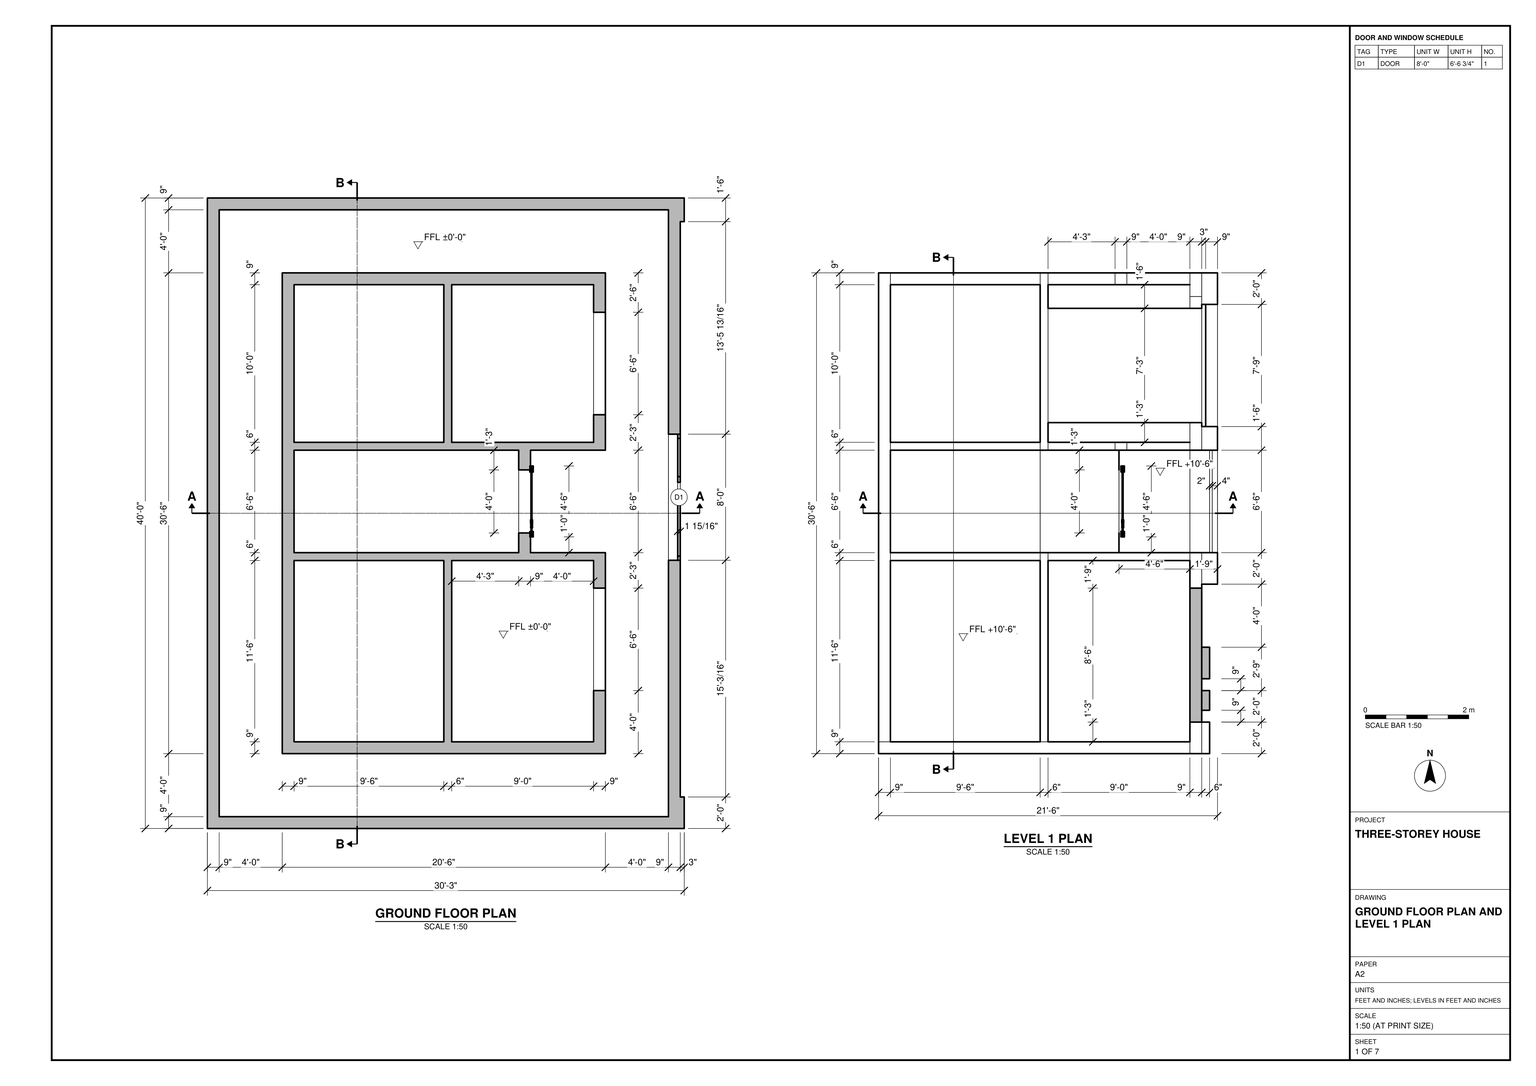
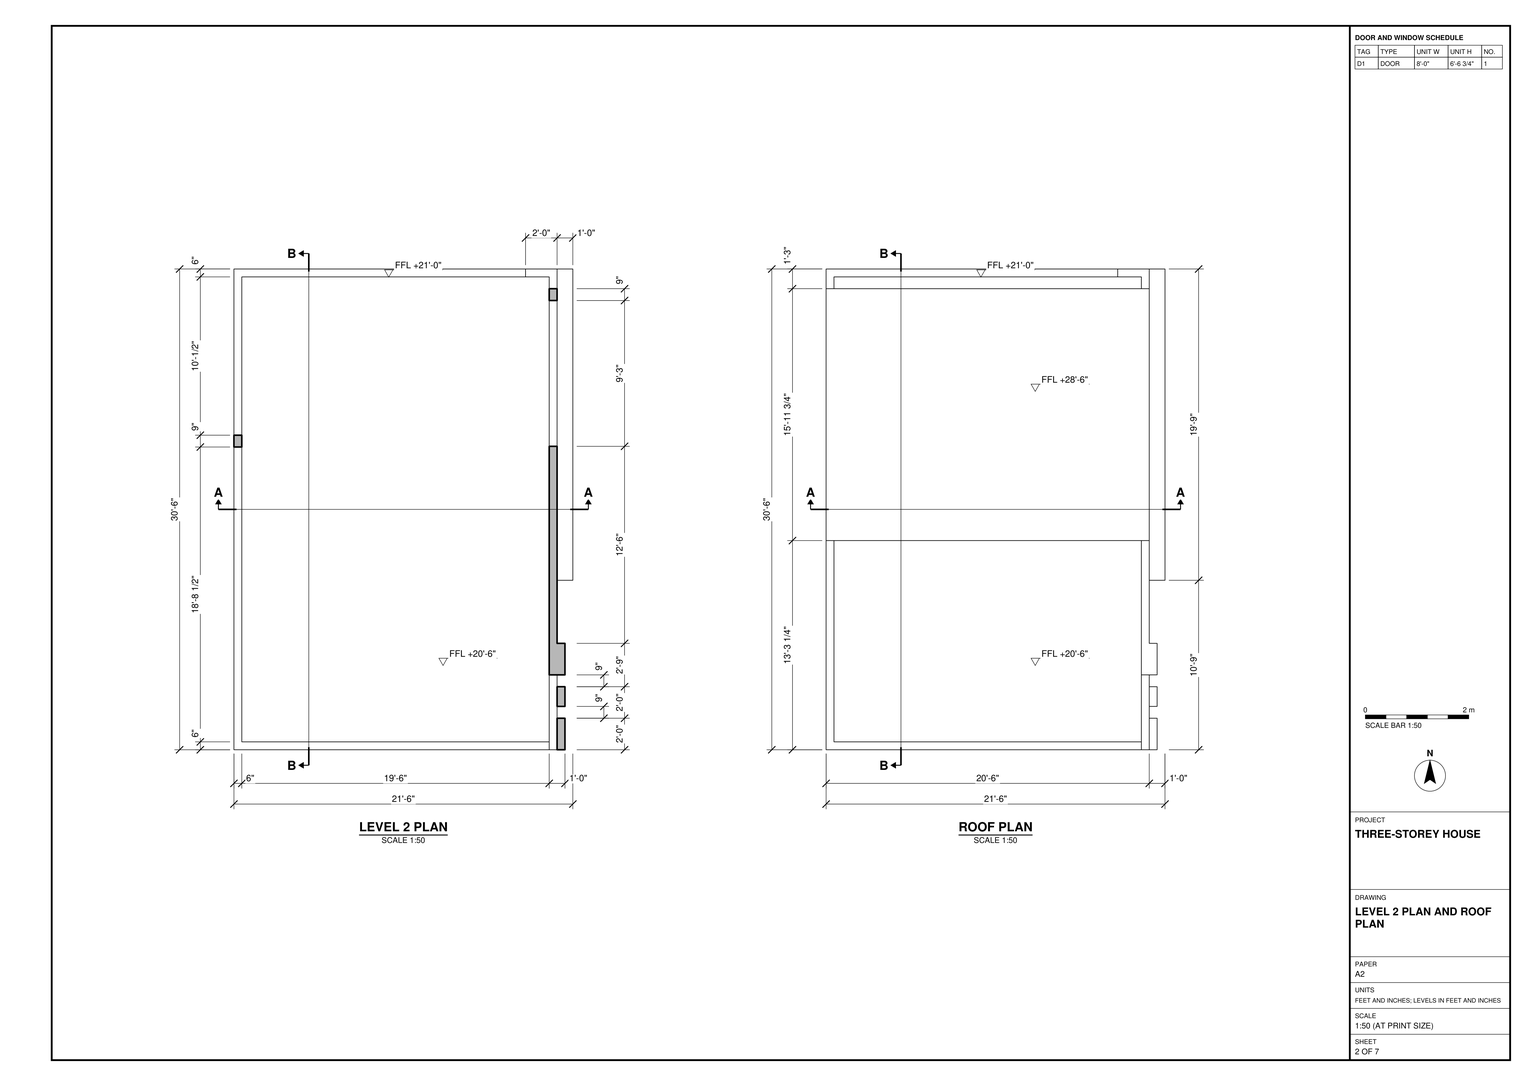
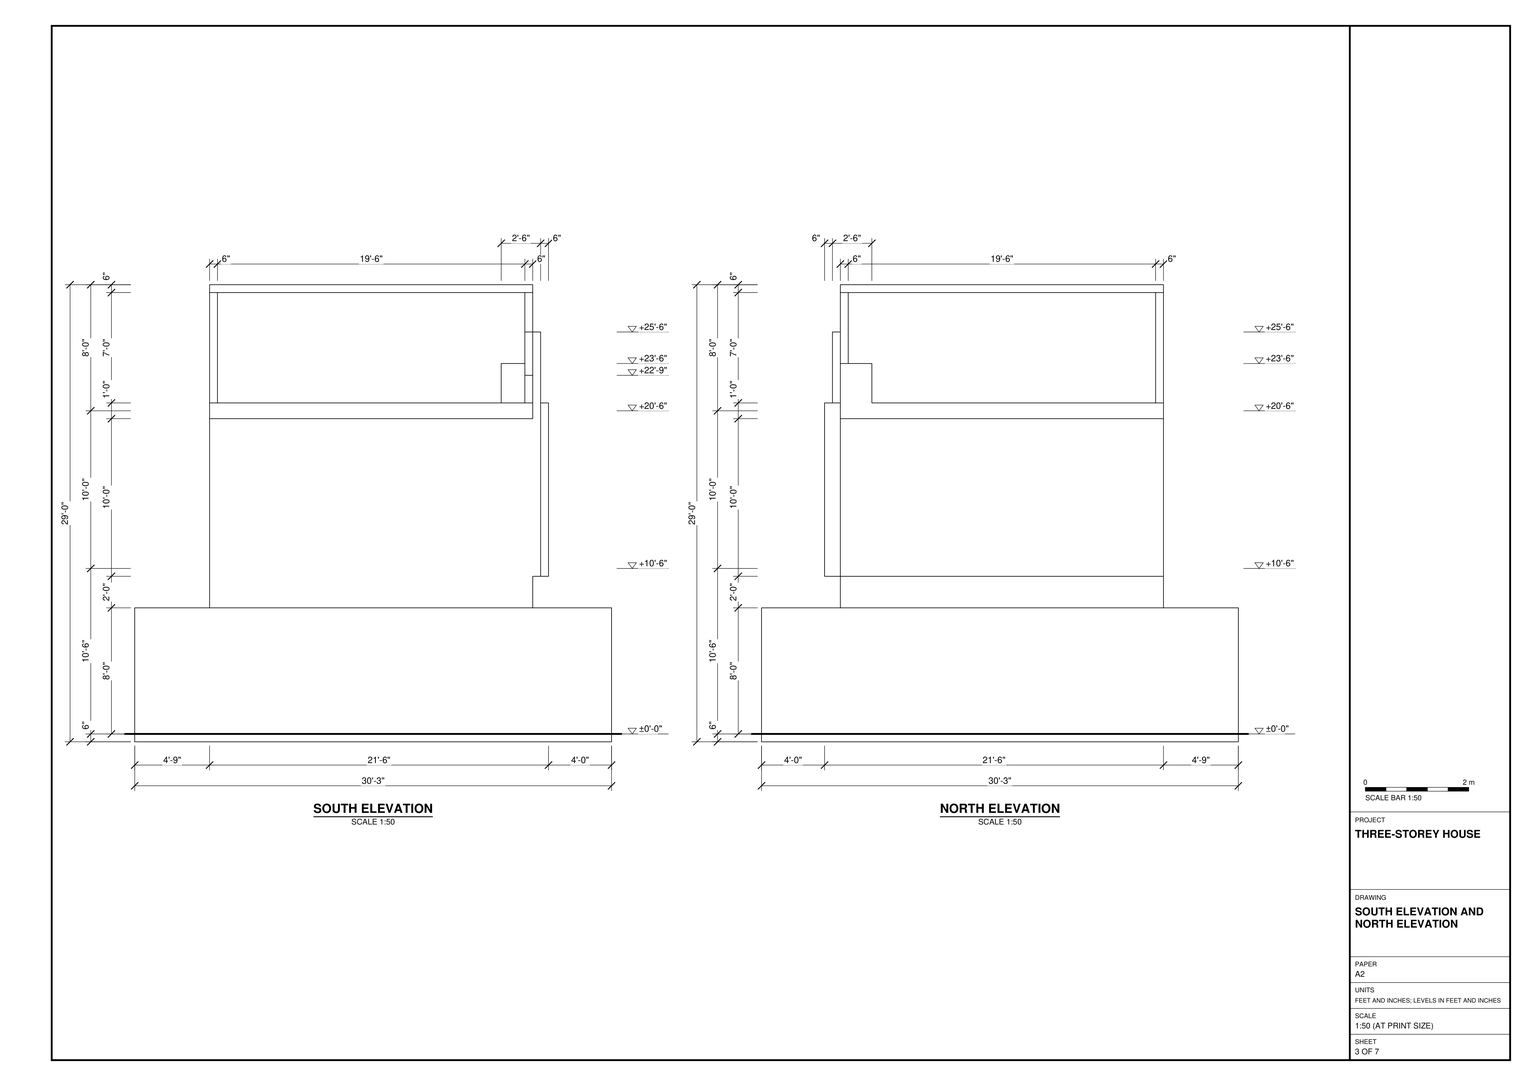
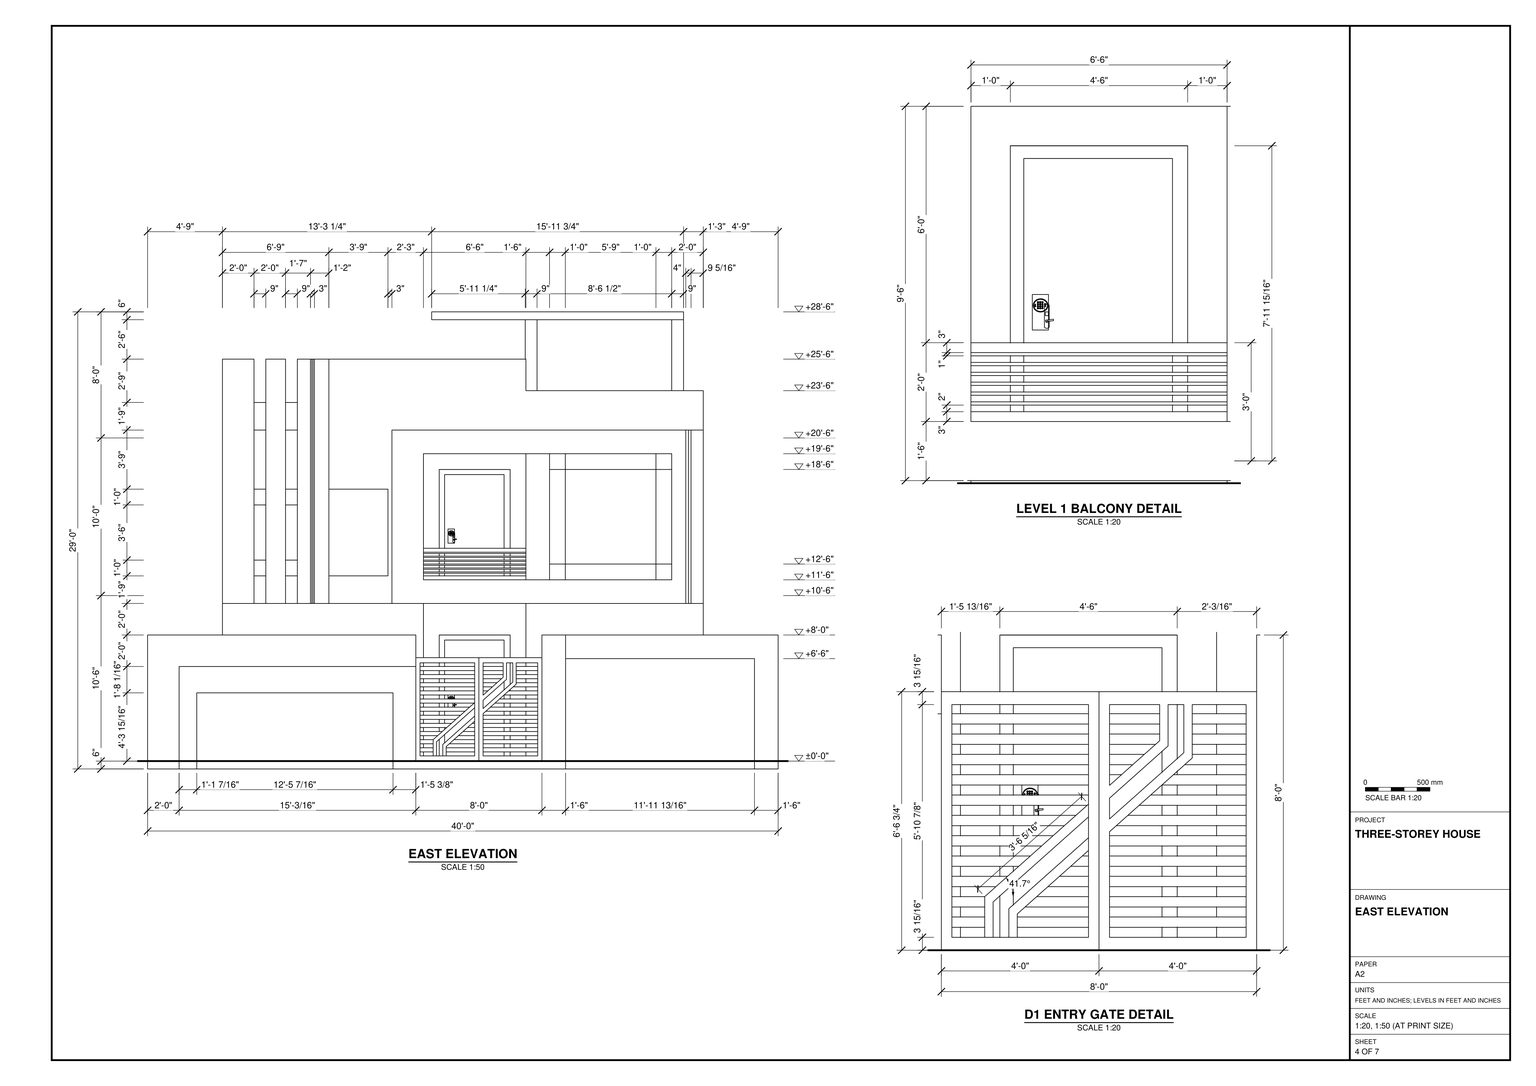
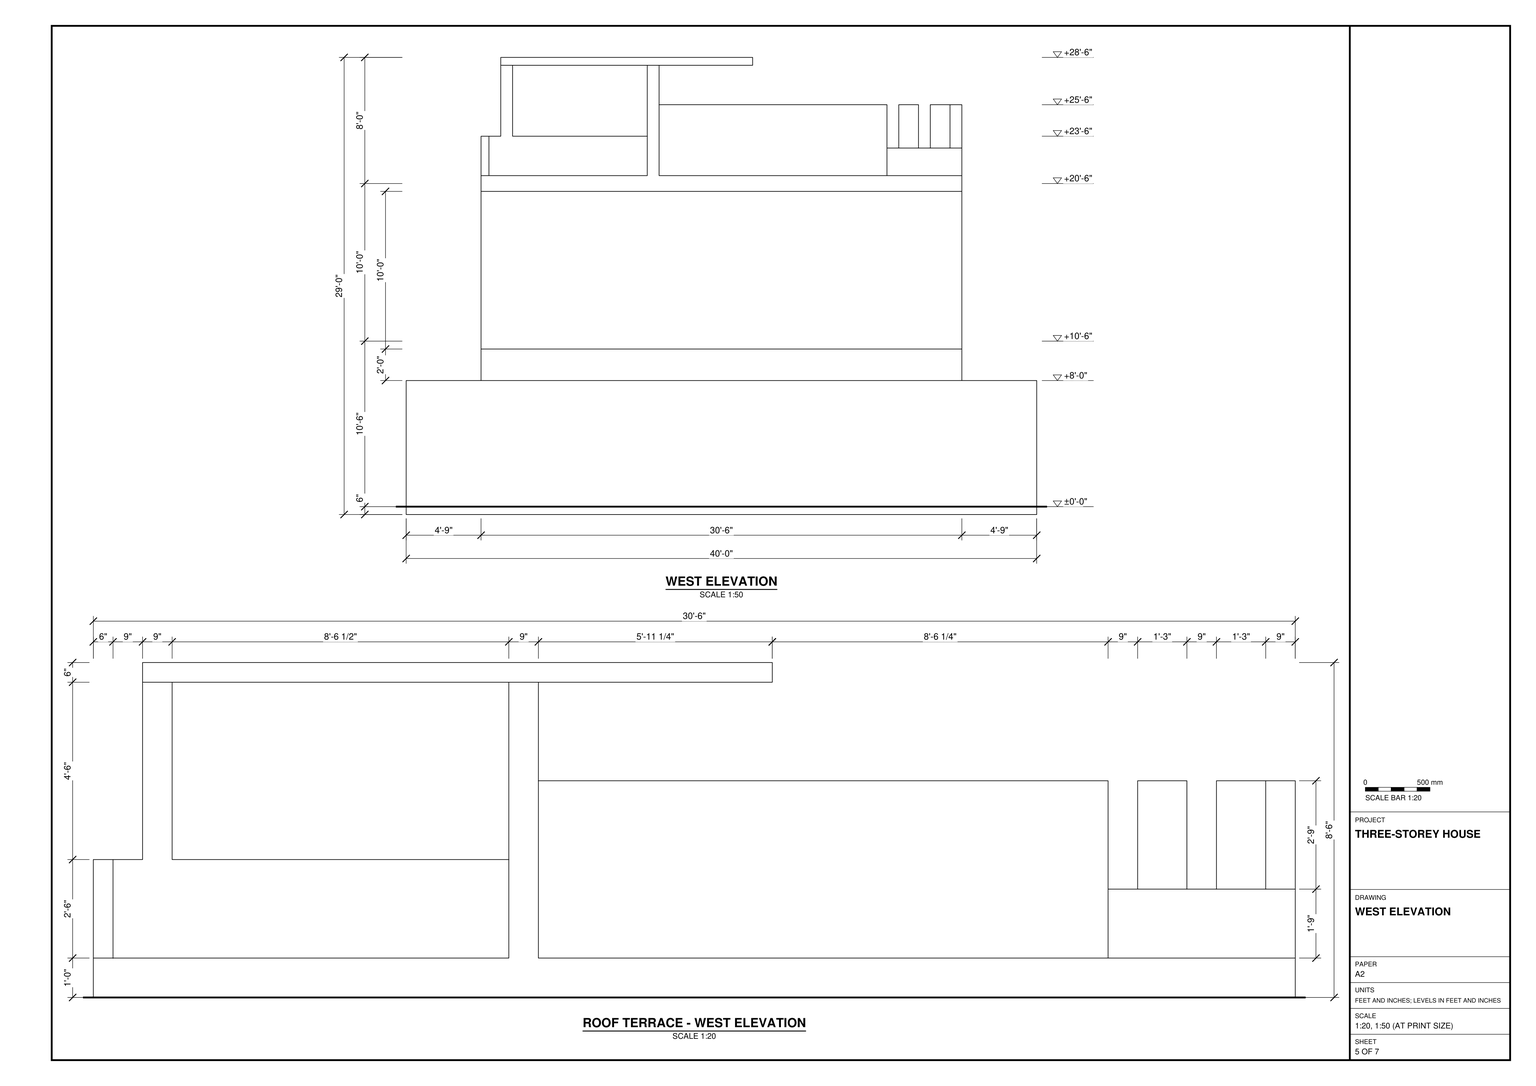
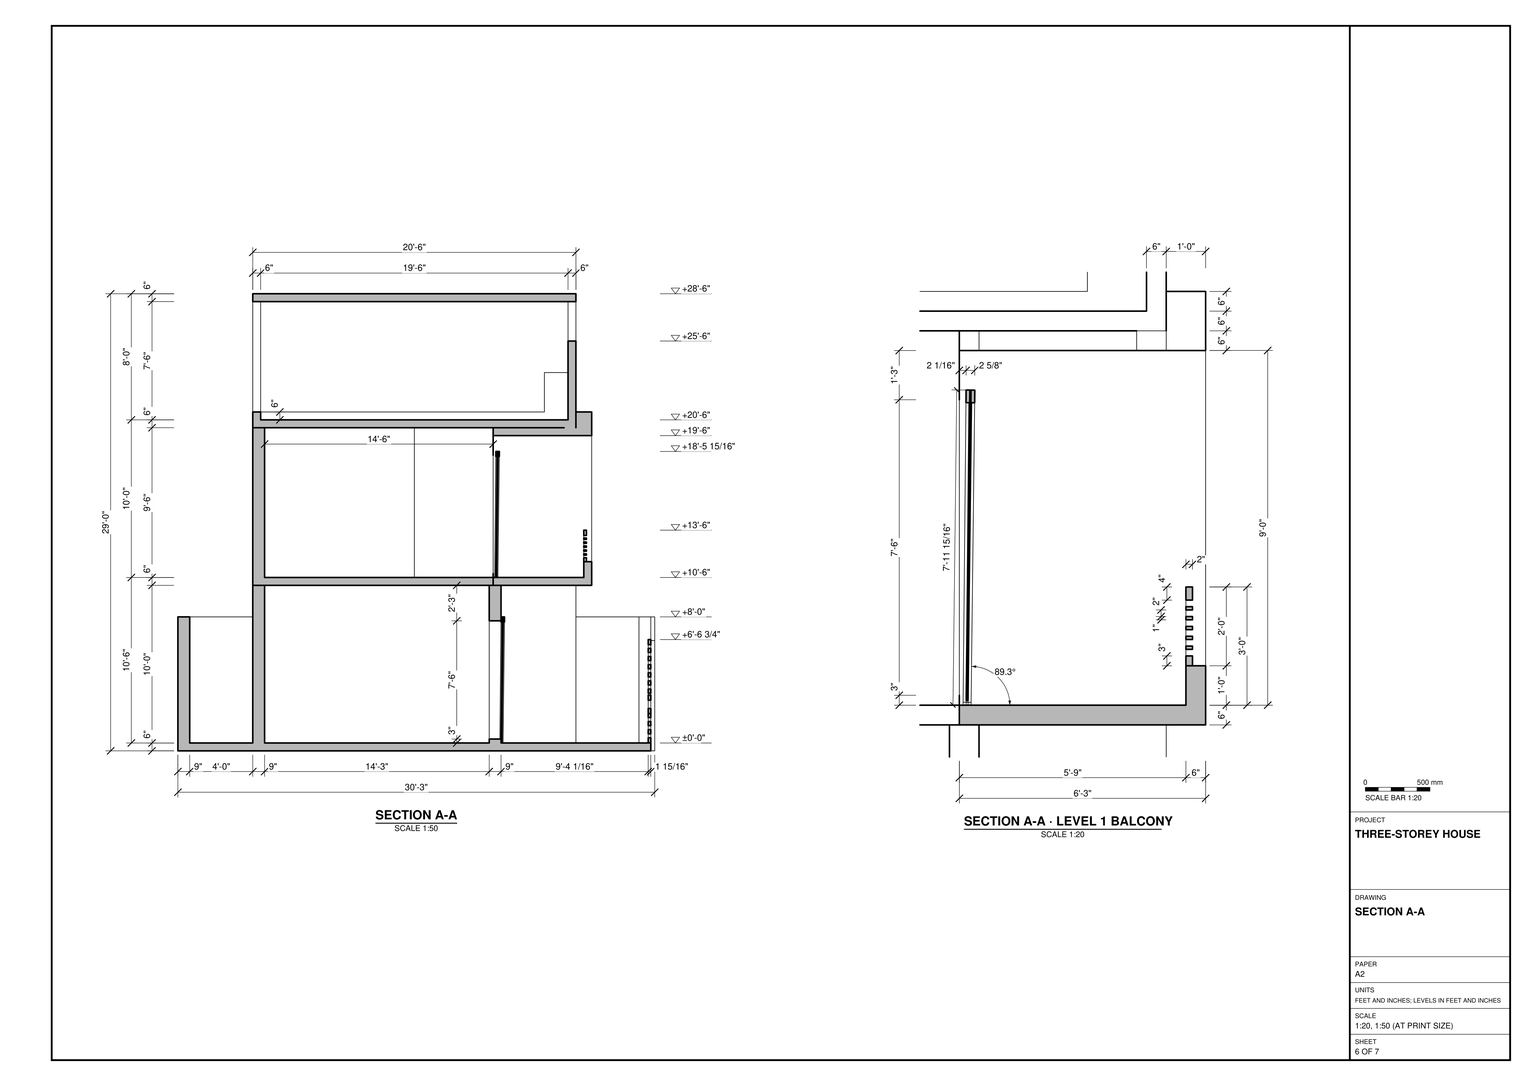
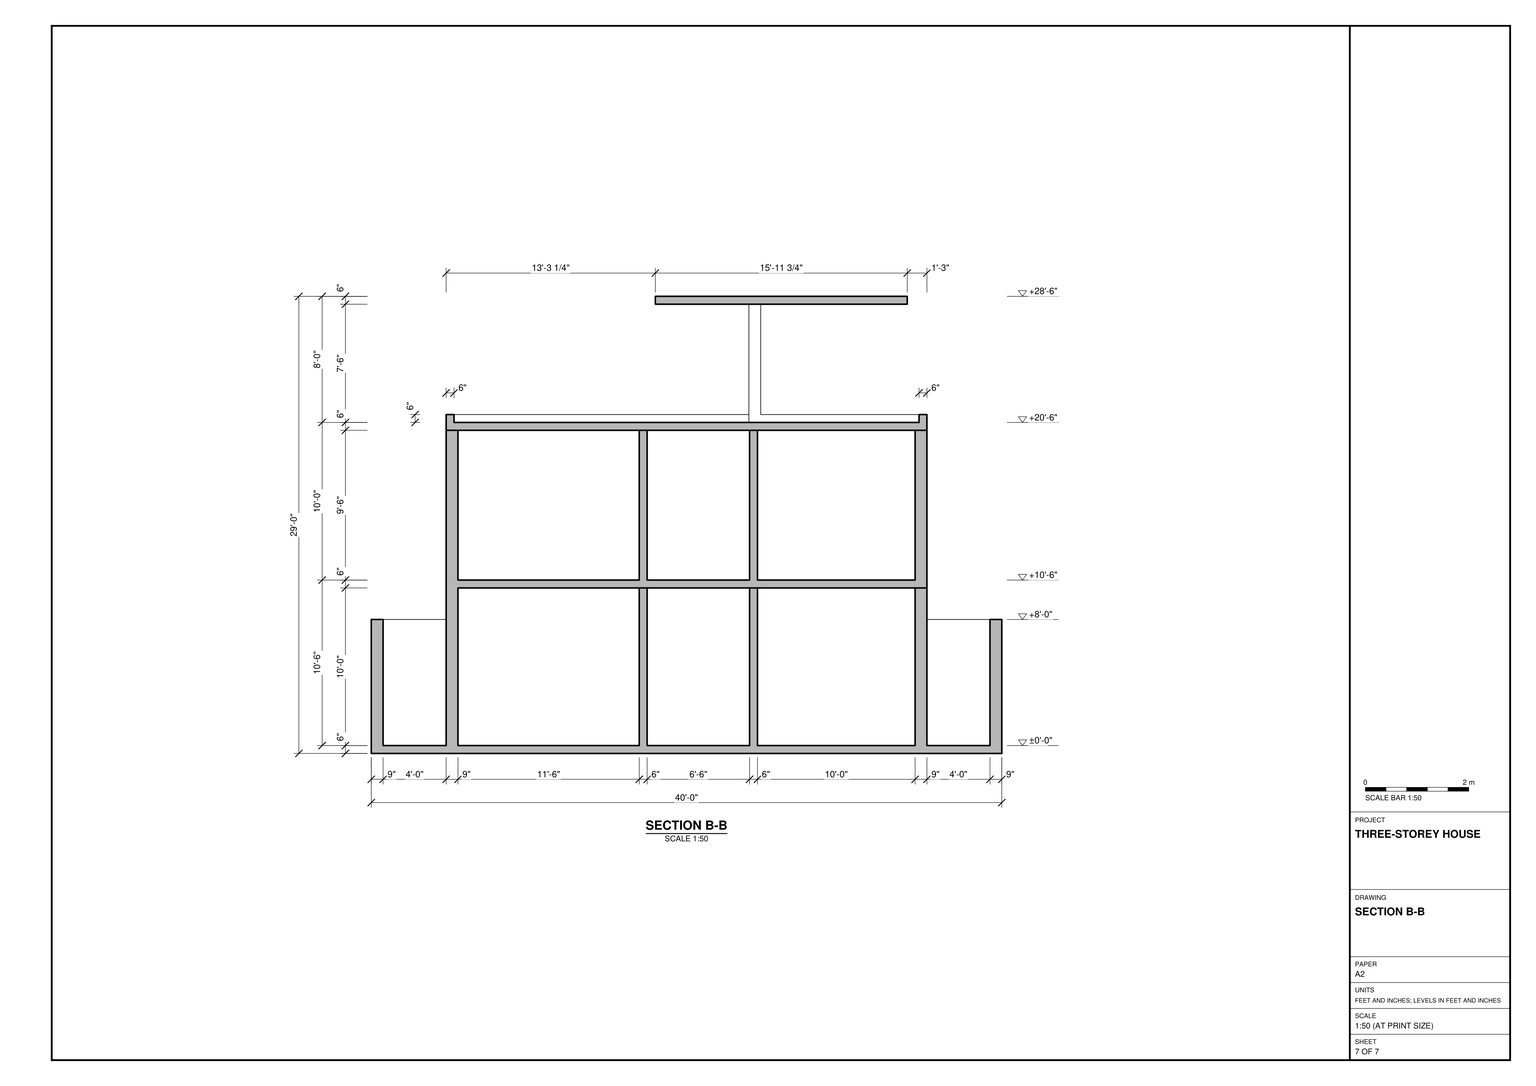
Build the three-storey house in SketchUp using task_files/diagram_01.pdf. Work in feet and inches. Orient the plan with the east entrance on the right. The overall model, including the perimeter enclosure, measures 30'-3" east to west, 40'-0" north to south and 29'-0" high. Set the floor levels at ±0'-0", +10'-6" and +20'-6".

Start with the rectangular perimeter wall and its entrance gate. Set the ground-floor shell inside the wall, leaving the clear strip around the house shown in plan. Lay out the paired rooms at the north and south ends and the central space between them. Follow the drawn wall thicknesses and distinguish the entrance through the perimeter wall from the openings in the east face of the house.

Model the floor slabs and the projecting sections of the east face at Level 1. At Level 2, extend the terrace across the footprint shown, then add the raised flat roof over the northern portion, leaving the southern portion uncovered. Use the elevations and sections to set the slab edges, roof supports and parapets.

Keep walls, slabs and roof elements in separate groups or components. Keep each furniture or joinery piece shown separate, and use components for repeated parts. Any decor or loose items shown may be suitable library components. Save one SketchUp model as output_files/gated_three_storey_house_with_roof_terrace.skp.

# SketchUp Ruby script. Lengths in inches.
U = 1.inch
M = Sketchup.active_model
def pt(a) = Geom::Point3d.new(a.map { |v| v * U })
def face(e, loops, mat)
  f = e.add_face(loops[0].map { |a| pt(a) })
  loops[1..].each { |l| e.add_face(l.map { |a| pt(a) }).erase! }
  f.material = f.back_material = mat if mat
  f
end
# faces: each face lists its corners as indices into pts; further lists are holes
def faces(e, pts, list, mat = nil) = list.each { |f| face(e, (f[0].is_a?(Array) ? f : [f]).map { |l| l.map { |i| pts[i] } }, mat) }
# xy, xz, yz: faces in a plane at the given z, y or x. An outline is a flat list of corners, or four numbers for a rectangle; further outlines are holes
def ring(l) = l.size == 4 ? [[l[0], l[1]], [l[2], l[1]], [l[2], l[3]], [l[0], l[3]]] : l.each_slice(2).to_a
def flat(e, list, mat, &to3) = list.each { |f| face(e, (f[0].is_a?(Array) ? f : [f]).map { |l| ring(l).map { |u, v| to3.(u, v) } }, mat) }
def xy(e, z, list, mat = nil) = flat(e, list, mat) { |x, y| [x, y, z] }
def xz(e, y, list, mat = nil) = flat(e, list, mat) { |x, z| [x, y, z] }
def yz(e, x, list, mat = nil) = flat(e, list, mat) { |y, z| [x, y, z] }
def lines(e, pts, list) = list.each { |a, b| e.add_line(pt(pts[a]), pt(pts[b])) }
# prism: a flat outline (further loops are holes) pulled along v
def prism(e, loops, v, mat = nil)
  f = face(e, loops, mat); d = Geom::Vector3d.new(v.map { |x| x * U })
  f.pushpull(f.normal.samedirection?(d) ? d.length : -d.length)
end
def box(e, o, s, mat = nil) = prism(e, [[o, [o[0] + s[0], o[1], o[2]], [o[0] + s[0], o[1] + s[1], o[2]], [o[0], o[1] + s[1], o[2]]]], [0, 0, s[2]], mat)
def at(x, y, z, deg = 0) = Geom::Transformation.translation(pt([x, y, z])) * Geom::Transformation.rotation(ORIGIN, Z_AXIS, deg.degrees)
def axes(o, x, y, z) = Geom::Transformation.new([*x, 0, *y, 0, *z, 0, *pt(o).to_a, 1])
def part(name) = M.definitions.add(name)
# library, detail: a bought-in or finely detailed component or shape, given as its bounding box
def library(name, o, s) = part(name).tap { |d| box(d.entities, o, s) }
def detail(e, o, s) = box(e.add_group.entities, o, s)
def put(e, d, t, mat = nil) = e.add_instance(d, t).tap { |i| i.material = mat if mat }
def group(e, t, mat = nil) = e.add_group.tap { |g| g.transformation = t; g.material = mat if mat }.entities
root = M.entities
M.materials.add("D04_Dandelion_Burst").color = [255, 204, 50]
M.materials.add("Glass_Basic_01").color = [255, 244, 143]
M.materials["Glass_Basic_01"].alpha = 0.25
M.materials.add("Glass_Basic_1").color = [161, 173, 186]
M.materials["Glass_Basic_1"].alpha = 0.25
M.materials.add("Marble_07_1K").color = [36, 34, 36]
M.materials.add("ThomThom - Buttons2").color = [40, 40, 43]
M.materials.add("ThomThom - Waistcoat2").color = [127, 127, 126]
M.materials.add("Wood_Veneer_15_1K").color = [103, 69, 45]
M.materials.add("[Wood_Cherry_Original]1").color = [76, 43, 21]
M.materials.add("[_0053_Ivory_]").color = [200, 200, 200]
M.materials.add("fabric_01").color = [251, 251, 251]
c1 = library("Modern+Gate+1",[0,0,0],[118.11,1.97,78.74])
c2 = library("porta+4",[0.2,-5.42,1.33],[46.55,4.72,83.21])
xy(root,273,[[297,57,303,114]])
xz(root,57,[[297,252,303,273]])
yz(root,297,[[57,252,114,273]])
yz(root,303,[[57,252,114,273]])
p = [[303,309,141],[303,396,141]]
lines(root,p,[[0,1]])
put(root,c1,axes([360,204.19,0],[0,0.8128,0],[-1,0,0],[0,0,1]))
g1 = group(root,at(0,0,0))
xy(g1,-6,[[0,0,0,480,363,480,363,462,360,462,360,24,363,24,363,0]])
xy(g1,0,[[[9,9,351,471],[57,57,57,423,303,423,303,288,246,288,246,210,303,210,303,57]],[66,66,180,204],[186,66,294,204],[351,204.19,360,300.19],[66,210,237,288],
  [66,294,180,414],[186,294,294,414]])
xy(g1,3,[[237,225,246,273]])
xy(g1,39,[[294,105,303,183],[294,315,303,393]])
xy(g1,72,[[360,24,363,204.19]])
xy(g1,78,[[360,318.19,363,462]])
xy(g1,93,[[294,105,303,183],[237,225,246,273],[294,315,303,393]])
xy(g1,96,[[0,0,363,0,363,204.19,351,204.19,351,9,9,9,9,471,351,471,351,300.19,360,300.19,360,318.19,363,318.19,363,480,0,480]])
xy(g1,120,[[303,57,309,81],[57,66,66,423],[66,66,180,204],[180,66,186,210],[186,66,294,204],
  [303,90,309,105],[303,114,309,138],[66,204,180,210],[186,204,294,204,294,210,240,210,240,288,246,288,246,294,237,294,237,210,186,210],[66,210,180,288],
  [180,210,186,288],[186,210,237,288],[240,210,246,288],[66,288,180,294],[180,288,186,423],
  [186,288,237,294],[246,288,294,294],[294,288,303,423],[66,294,180,414],[186,294,237,414],
  [237,294,246,414],[246,294,294,414],[66,414,180,423],[186,414,237,423],[237,414,246,423],
  [246,414,294,423]])
xy(g1,120,[[303,186,315,210],[303,288,315,423]],"ThomThom - Waistcoat2")
xy(g1,120,[[246,210,315,288]],"[_0053_Ivory_]")
xy(g1,126,[[66,66,180,204],[186,66,294,204],[66,210,180,288],[180,210,240,288],[240,210,294,288],
  [294,210,309,288],[66,294,180,414],[186,294,294,414]])
xy(g1,138,[[303,306,306,399]])
xy(g1,138,[[309,210,311,288],[311,210,315,288],[306,306,315,399]],"ThomThom - Waistcoat2")
xy(g1,141,[[294,81,303,183],[309,210,311,288],[186,309,303,396]])
xy(g1,143,[[309,210,311,288]])
xy(g1,144,[[309,210,311,288]])
xy(g1,146,[[309,210,311,288]])
xy(g1,147,[[309,210,311,288]])
xy(g1,149,[[309,210,311,288]])
xy(g1,150,[[309,210,311,288]])
xy(g1,152,[[309,210,311,288]])
xy(g1,153,[[309,210,311,288]])
xy(g1,155,[[309,210,311,288]])
xy(g1,156,[[309,210,311,288]])
xy(g1,158,[[309,210,311,288]])
xy(g1,162,[[309,210,311,288]],"ThomThom - Buttons2")
xy(g1,207,[[294,81,303,183]])
xy(g1,231,[[186,309,303,396]])
xy(g1,234,[[240,210,315,288],[303,306,306,399],[306,306,315,399]],"[_0053_Ivory_]")
xy(g1,240,[[57,57,66,423],[66,57,180,66],[180,57,186,210],[186,57,240,66],[240,57,246,66],
  [246,57,294,66],[66,66,180,204],[186,66,240,204],[240,66,246,204],[246,66,294,204],
  [66,204,180,210],[186,204,240,210],[240,204,246,204,246,288,294,288,294,294,186,294,186,288,240,288],[246,204,294,210],[66,210,180,288],
  [180,210,186,288],[186,210,240,288],[246,210,294,288],[66,288,180,294],[180,288,186,423],
  [294,288,303,294],[66,294,180,414],[186,294,294,414],[294,294,303,423],[66,414,180,423],
  [186,414,294,423]])
xy(g1,246,[[63,63,297,417]],"fabric_01")
xy(g1,252,[[57,57,303,57,303,114,297,114,297,63,63,63,63,287.48,57,287.48],[57,296.48,63,296.48,63,417,279,417,279,423,57,423]])
xy(g1,252,[[303,186,315,423]],"ThomThom - Waistcoat2")
xy(g1,282,[[297,288,303,399],[297,408,303,408,303,423,279,423,279,417,297,417]])
xy(g1,306,[[303,57,309,81],[303,90,309,105],[297,114,309,114,309,138,303,138,303,288,297,288]])
xy(g1,336,[[57,287.48,63,296.48],[297,399,303,408]])
xy(g1,336,[[[81,237.625,279,384],[85,241.625,275,311.48],[85,315.48,275,380]]],"D04_Dandelion_Burst")
xy(g1,336,[[57,216.25,63,287.48],[[63,216.25,63,296.48,57,296.48,57,408,297,408,297,399,303,399,303,216.25],[81,237.625,279,384]],[85,241.625,275,311.48],[85,315.48,275,380]],"Wood_Veneer_15_1K")
xy(g1,342,[[57,216.25,303,408]],"Wood_Veneer_15_1K")
xz(g1,0,[[0,-6,363,96]],"fabric_01")
xz(g1,9,[[9,0,351,96]])
xz(g1,24,[[360,-6,363,72]])
xz(g1,57,[[57,240,303,252]])
xz(g1,57,[[57,0,303,0,303,120,309,120,309,306,303,306,303,240,57,240]],"fabric_01")
xz(g1,63,[[63,246,297,252]])
xz(g1,66,[[66,0,180,120],[186,0,294,120],[66,126,180,240],[186,126,294,240]])
xz(g1,81,[[303,120,309,306],[294,141,303,207]])
xz(g1,90,[[303,120,309,306]])
xz(g1,105,[[294,39,303,93],[303,120,309,306]])
xz(g1,114,[[303,120,309,120,309,306,297,306,297,252,303,252]])
xz(g1,138,[[303,120,309,306]])
xz(g1,183,[[294,39,303,93],[294,141,303,207]])
xz(g1,186,[[303,120,315,252]],"ThomThom - Waistcoat2")
xz(g1,204,[[66,0,180,120],[186,0,294,120],[66,126,180,240],[186,126,294,240]])
xz(g1,204.19,[[351,0,351,96,363,96,363,72,360,72,360,0]])
xz(g1,210,[[66,0,237,120],[240,120,294,126],[66,126,180,240],[180,126,240,240],[246,234,294,240]])
xz(g1,210,[[246,0,303,120],[[240,126,240,234,315,234,315,138,311,138,311,141,309,141,309,126],[309,158,311,162],[309,155,311,156],[309,152,311,153],[309,149,311,150],[309,146,311,147],[309,143,311,144]],[309,138,311,141],[309,143,311,144],[309,146,311,147],
  [309,149,311,150],[309,152,311,153],[309,155,311,156],[309,158,311,162]],"[_0053_Ivory_]")
xz(g1,216.25,[[57,336,303,342]],"Wood_Veneer_15_1K")
xz(g1,225,[[237,3,246,93]])
xz(g1,273,[[237,3,246,93]])
xz(g1,287.48,[[57,252,63,336]])
xz(g1,288,[[66,0,237,120],[240,120,294,126],[66,126,180,240],[180,126,240,240],[246,234,294,240],
  [297,282,303,306]])
xz(g1,288,[[246,0,303,120],[[240,126,309,126,309,141,311,141,311,138,315,138,315,234,240,234],[309,158,311,162],[309,155,311,156],[309,152,311,153],[309,149,311,150],[309,146,311,147],[309,143,311,144]],[309,138,311,141],[309,143,311,144],[309,146,311,147],
  [309,149,311,150],[309,152,311,153],[309,155,311,156],[309,158,311,162]],"[_0053_Ivory_]")
xz(g1,294,[[66,0,180,120],[186,0,294,120],[66,126,180,240],[186,126,294,240]])
xz(g1,296.48,[[57,252,63,336]])
xz(g1,300.19,[[351,0,360,96]])
xz(g1,306,[[303,138,306,234],[306,138,315,234]])
xz(g1,309,[[186,141,303,231]])
xz(g1,315,[[294,39,303,93]])
xz(g1,318.19,[[360,78,363,96]])
xz(g1,393,[[294,39,303,93]])
xz(g1,396,[[186,141,303,231]])
xz(g1,399,[[297,282,303,336]])
xz(g1,399,[[303,138,306,234],[306,138,315,234]],"ThomThom - Waistcoat2")
xz(g1,408,[[297,282,303,336]])
xz(g1,408,[[57,336,303,342]],"Wood_Veneer_15_1K")
xz(g1,414,[[66,0,180,120],[186,0,294,120],[66,126,180,240],[186,126,294,240]])
xz(g1,417,[[63,246,297,246,297,282,279,282,279,252,63,252]],"fabric_01")
xz(g1,423,[[57,240,57,252,279,252,279,282,303,282,303,240]])
xz(g1,423,[[303,120,315,252]],"ThomThom - Waistcoat2")
xz(g1,423,[[57,0,303,120],[57,120,303,240]],"fabric_01")
xz(g1,462,[[360,-6,363,78]])
xz(g1,471,[[9,0,351,96]])
xz(g1,480,[[0,-6,363,96]],"fabric_01")
yz(g1,0,[[0,-6,480,96]],"fabric_01")
yz(g1,9,[[9,0,471,96]])
yz(g1,57,[[57,240,57,252,287.48,252,287.48,336,296.48,336,296.48,252,423,252,423,240]])
yz(g1,57,[[216.25,336,408,342]],"Wood_Veneer_15_1K")
yz(g1,57,[[57,0,423,120],[57,120,423,240]],"fabric_01")
yz(g1,63,[[63,246,287.48,252],[287.48,246,417,246,417,252,296.48,252,296.48,336,287.48,336]])
yz(g1,66,[[66,0,204,120],[210,0,288,120],[294,0,414,120],[66,126,204,240],[210,126,288,240],
  [294,126,414,240]])
yz(g1,180,[[66,0,204,120],[294,0,414,120],[66,126,204,240],[294,126,414,240]])
yz(g1,186,[[66,0,204,120],[294,0,414,120],[66,126,204,240],[[294,126,414,240],[309,141,396,231]]])
yz(g1,237,[[[210,0,288,120],[225,3,273,93]]])
yz(g1,240,[[210,120,222,126],[222,120,276,120,276,126,273,126,273,123,225,123,225,126,222,126],[276,120,288,126],[225,123,273,126],[[222,126,276,222],[225,129,273,219]],
  [210,234,288,240]])
yz(g1,240,[[210,126,222,126,222,222,276,222,276,126,288,126,288,234,210,234]],"[_0053_Ivory_]")
yz(g1,246,[[[222,0,276,96],[225,3,273,93]]])
yz(g1,246,[[210,0,222,0,222,96,276,96,276,0,288,0,288,120,210,120]],"[_0053_Ivory_]")
yz(g1,279,[[417,252,423,282]])
yz(g1,294,[[[66,0,204,120],[105,39,183,93]],[[294,0,414,120],[315,39,393,93]],[66,126,66,240,186,240,186,210,78,210,78,138,186,138,186,126],[186,126,204,240],[[78,138,186,210],[81,141,183,207]]])
yz(g1,294,[[81,141,183,207]],"Glass_Basic_01")
yz(g1,297,[[63,246,114,252],[288,246,294,282]])
yz(g1,297,[[114,246,288,306],[294,246,294,282,399,282,399,336,408,336,408,282,417,282,417,246]],"fabric_01")
yz(g1,303,[[315,39,393,41.68],[90,120,105,141],[114,120,138,141],[[306,138,399,234],[309,141,396,231]],[90,141,93,153],
  [93,141,96,153],[96,141,105,153],[114,141,138,207],[90,153,93,195],[93,153,96,195],
  [96,153,105,195],[90,195,93,207],[93,195,96,207],[96,195,105,207],[90,207,93,240],
  [93,207,96,240],[96,207,105,240],[114,207,138,240],[57,240,81,252],[90,240,93,252],
  [93,240,96,252],[96,240,105,252],[114,240,138,273],[186,240,210,252],[210,240,288,252],
  [288,240,294,252],[294,240,423,252],[57,252,66,306],[93,252,96,273],[399,282,408,336]])
yz(g1,303,[[81,141,90,153],[105,141,114,153],[138,141,183,207],[81,153,90,195],[105,153,114,195],
  [81,195,90,207],[105,195,114,207]],"Glass_Basic_01")
yz(g1,303,[[105,39,183,93],[315,41.68,393,93]],"Glass_Basic_1")
yz(g1,303,[[81,207,90,252],[105,207,114,252]],"Marble_07_1K")
yz(g1,303,[[216.25,336,408,342]],"Wood_Veneer_15_1K")
yz(g1,303,[[[102,36,186,96],[105,39,183,93]],[[312,36,396,96],[315,39,393,93]]],"[Wood_Cherry_Original]1")
yz(g1,303,[[[57,0,210,120],[102,36,186,96]],[[288,0,423,120],[312,36,396,96]],[81,120,90,141],[105,120,114,141],[138,120,186,120,186,252,423,252,423,282,288,282,288,306,138,306,138,207,183,207,183,141,138,141],
  [66,252,81,306],[90,252,90,306,105,306,105,273,93,273,93,252],[96,252,105,273]],"fabric_01")
yz(g1,306,[[306,138,318,150],[318,138,387,150],[387,138,399,150],[306,150,318,222],[318,150,387,222],
  [387,150,399,222],[306,222,318,234],[318,222,387,234],[387,222,399,234]],"Glass_Basic_01")
yz(g1,309,[[125,120,126,306],[210,126,288,138],[210,138,288,141],[210,143,288,144],[210,146,288,147],
  [210,149,288,150],[210,152,288,153],[210,155,288,156],[210,158,288,162]])
yz(g1,309,[[124,120,125,306],[126,120,127,306]],"[_0053_Ivory_]")
yz(g1,309,[[57,120,81,306],[90,120,105,306],[114,120,124,306],[127,120,138,306]],"fabric_01")
yz(g1,311,[[210,138,288,141],[210,143,288,144],[210,146,288,147],[210,149,288,150],[210,152,288,153],
  [210,155,288,156],[210,158,288,159],[210,159,288,162]],"ThomThom - Buttons2")
yz(g1,315,[[[186,120,409.7,252],[210,138,399,234]]],"Marble_07_1K")
yz(g1,315,[[413.7,120,423,252]],"ThomThom - Waistcoat2")
yz(g1,315,[[409.7,120,411.7,252],[411.7,120,413.7,252]],"[_0053_Ivory_]")
yz(g1,315,[[288,138,306,234]],"fabric_01")
yz(g1,351,[[9,0,204.19,96],[300.19,0,471,96]])
yz(g1,360,[[37.42,-6,186.83,51.95]],"Marble_07_1K")
yz(g1,360,[[24,-6,37.42,-6,37.42,51.95,186.83,51.95,186.83,-6,318.19,-6,318.19,96,300.19,96,300.19,0,204.19,0,204.19,72,24,72],[318.19,-6,462,78]],"fabric_01")
yz(g1,363,[[0,-6,24,-6,24,72,204.19,72,204.19,96,0,96],[462,-6,480,-6,480,96,318.19,96,318.19,78,462,78]],"fabric_01")
p = [[294,204,0],[294,210,0],[294,288,0],[294,294,0],[294,66,120],[294,57,120],
  [294,288,126],[294,294,126],[294,204,126],[294,210,126],[294,312,138],[294,312,141],
  [294,405,138],[294,405,222],[303,312,138],[303,405,138],[303,405,222],[303,114,273],
  [303,105,273],[309,210,156],[309,210,158],[309,288,158],[309,288,156],[309,210,153],
  [309,210,155],[309,288,155],[309,288,153],[309,210,150],[309,210,152],[309,288,152],
  [309,288,150],[309,210,147],[309,210,149],[309,288,149],[309,288,147],[309,210,144],
  [309,210,146],[309,288,146],[309,288,144],[309,210,141],[309,210,143],[309,288,143],
  [309,288,141]]
lines(g1,p,[[0,1],[2,3],[4,5],[6,7],[8,9],[10,11],[10,12],[12,13],[14,10],[15,12],[16,13],[17,18],
  [19,20],[21,22],[23,24],[25,26],[27,28],[29,30],[31,32],[33,34],[35,36],[37,38],[39,40],[41,42]])
put(g1,c2,axes([239.3,221.77,124.46],[0,1.16008,0],[-1,0,0],[0,0,1.15383]))
put(g1,c2,axes([243.24,221.77,-1.54],[0,1.16008,0],[-1,0,0],[0,0,1.15408]))
